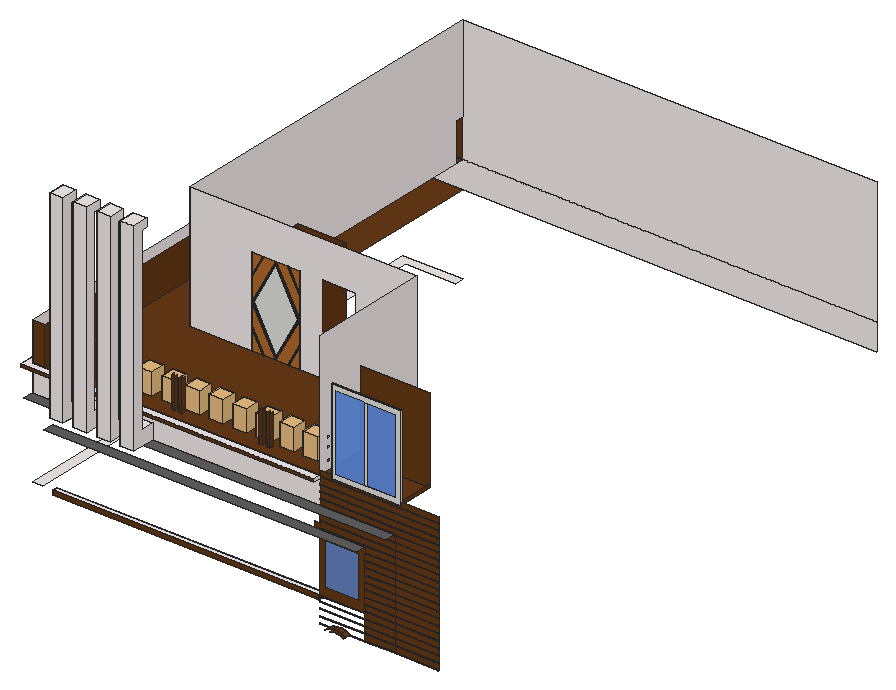
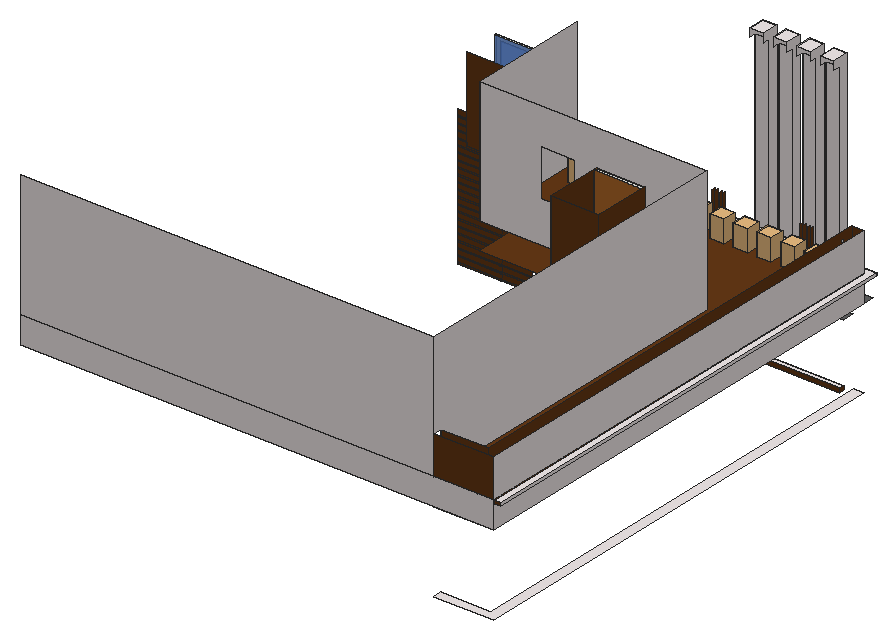
# SketchUp Ruby script. Lengths in inches.
U = 1.inch
M = Sketchup.active_model
def pt(a) = Geom::Point3d.new(a.map { |v| v * U })
def face(e, loops, mat)
  f = e.add_face(loops[0].map { |a| pt(a) })
  loops[1..].each { |l| e.add_face(l.map { |a| pt(a) }).erase! }
  f.material = f.back_material = mat if mat
  f
end
# faces: each face lists its corners as indices into pts; further lists are holes
def faces(e, pts, list, mat = nil) = list.each { |f| face(e, (f[0].is_a?(Array) ? f : [f]).map { |l| l.map { |i| pts[i] } }, mat) }
# xy, xz, yz: faces in a plane at the given z, y or x. An outline is a flat list of corners, or four numbers for a rectangle; further outlines are holes
def ring(l) = l.size == 4 ? [[l[0], l[1]], [l[2], l[1]], [l[2], l[3]], [l[0], l[3]]] : l.each_slice(2).to_a
def flat(e, list, mat, &to3) = list.each { |f| face(e, (f[0].is_a?(Array) ? f : [f]).map { |l| ring(l).map { |u, v| to3.(u, v) } }, mat) }
def xy(e, z, list, mat = nil) = flat(e, list, mat) { |x, y| [x, y, z] }
def xz(e, y, list, mat = nil) = flat(e, list, mat) { |x, z| [x, y, z] }
def yz(e, x, list, mat = nil) = flat(e, list, mat) { |y, z| [x, y, z] }
def lines(e, pts, list) = list.each { |a, b| e.add_line(pt(pts[a]), pt(pts[b])) }
# prism: a flat outline (further loops are holes) pulled along v
def prism(e, loops, v, mat = nil)
  f = face(e, loops, mat); d = Geom::Vector3d.new(v.map { |x| x * U })
  f.pushpull(f.normal.samedirection?(d) ? d.length : -d.length)
end
def box(e, o, s, mat = nil) = prism(e, [[o, [o[0] + s[0], o[1], o[2]], [o[0] + s[0], o[1] + s[1], o[2]], [o[0], o[1] + s[1], o[2]]]], [0, 0, s[2]], mat)
def at(x, y, z, deg = 0) = Geom::Transformation.translation(pt([x, y, z])) * Geom::Transformation.rotation(ORIGIN, Z_AXIS, deg.degrees)
def axes(o, x, y, z) = Geom::Transformation.new([*x, 0, *y, 0, *z, 0, *pt(o).to_a, 1])
def part(name) = M.definitions.add(name)
# library, detail: a bought-in or finely detailed component or shape, given as its bounding box
def library(name, o, s) = part(name).tap { |d| box(d.entities, o, s) }
def detail(e, o, s) = box(e.add_group.entities, o, s)
def put(e, d, t, mat = nil) = e.add_instance(d, t).tap { |i| i.material = mat if mat }
def group(e, t, mat = nil) = e.add_group.tap { |g| g.transformation = t; g.material = mat if mat }.entities
root = M.entities
M.materials.add("Generic").color = [102, 57, 22]
M.materials.add("Generic\#1").color = [96, 96, 96]
M.materials.add("Generic\#3").color = [243, 235, 235]
M.materials.add("[Color M08]").color = [30, 30, 30]
M.materials.add("[Translucent Glass Blue]").color = [100, 149, 237]
M.materials["[Translucent Glass Blue]"].alpha = 0.79
M.materials.add("[Translucent Glass Blue]1").color = [100, 149, 237]
M.materials["[Translucent Glass Blue]1"].alpha = 0.5
M.materials.add("[Wood Bamboo]").color = [177, 105, 43]
c1 = part("Group\#5")
xy(c1.entities,0,[[0,0,33.5625,3]],"[Wood Bamboo]")
xy(c1.entities,44.875,[[0,0,33.5625,3]],"[Wood Bamboo]")
xz(c1.entities,0,[[3.04,3.04,15.78,41.84],[17.78,3.04,30.53,41.84]],"[Translucent Glass Blue]1")
xz(c1.entities,0,[[[0,0,33.5625,44.875],[3.04,3.04,15.78,41.84],[17.78,3.04,30.53,41.84]]],"[Wood Bamboo]")
xz(c1.entities,3,[[0,0,33.5625,44.875]],"[Translucent Glass Blue]1")
yz(c1.entities,0,[[0,0,3,44.875]],"[Wood Bamboo]")
yz(c1.entities,33.5625,[[0,0,3,44.875]],"[Wood Bamboo]")
c2 = part("Group\#3")
xy(c2.entities,14.5,[[0,9,13.0625,22.4375]])
xy(c2.entities,193.75,[[0,0,13.0625,15.5]])
xz(c2.entities,0,[[0,0,13.0625,193.75]])
xz(c2.entities,9,[[0,14.5,13.0625,185.625]])
yz(c2.entities,0,[[0,0,0,193.75,15.5,193.75,15.5,185.625,9,185.625,9,14.5,22.4375,14.5,22.4375,0]])
yz(c2.entities,13.0625,[[0,0,22.4375,0,22.4375,14.5,9,14.5,9,185.625,15.5,185.625,15.5,193.75,0,193.75]])
c3 = library("Raised potted plant",[1.65,0,0],[13.63,13.63,20.73])
c4 = part("Group\#4")
xy(c4.entities,0,[[10.55,0,10.55,0.4375,0,0.4375,0,3.4375,46.1875,3.4375,46.1875,0.4375,35.64,0.4375,35.64,0,34.64,0,34.64,0.4375,11.55,0.4375,11.55,0]])
xy(c4.entities,84.6875,[[11,0,11.55,0,11.55,0.4375,34.64,0.4375,34.64,0,35.1875,0,35.1875,0.4375,46.1875,0.4375,46.1875,3.4375,0,3.4375,0,0.4375,11,0.4375]])
xz(c4.entities,0,[[10.55,0,11.55,0,0,21.17,0,19.34],[[23.09,0,46.1875,42.34,23.09,84.6875,0,42.34],[23.09,2.875,1.57,42.34,23.09,81.8125,44.62,42.34]],[34.64,0,35.64,0,46.1875,19.34,46.1875,21.17],[0,63.52,11.55,84.6875,11,84.6875,0,64.52],[46.1875,63.52,46.1875,64.52,35.1875,84.6875,34.64,84.6875]],"[Color M08]")
xz(c4.entities,0.4375,[[23.09,2.875,44.62,42.34,23.09,81.8125,1.57,42.34]])
xz(c4.entities,0.4375,[[0,0,10.55,0,0,19.34],[11.55,0,23.09,0,0,42.34,0,21.17],[23.09,0,34.64,0,46.1875,21.17,46.1875,42.34],[35.64,0,46.1875,0,46.1875,19.34],[0,42.34,23.09,84.6875,11.55,84.6875,0,63.52],
  [46.1875,42.34,46.1875,63.52,34.64,84.6875,23.09,84.6875],[0,64.52,11,84.6875,0,84.6875],[46.1875,64.52,46.1875,84.6875,35.1875,84.6875]],"[Wood Bamboo]")
xz(c4.entities,3.4375,[[0,0,46.1875,84.6875]],"[Wood Bamboo]")
yz(c4.entities,0,[[0.4375,0,0.4375,19.34,0,19.34,0,21.17,0.4375,21.17,0.4375,63.52,0,63.52,0,64.52,0.4375,64.52,0.4375,84.6875,3.4375,84.6875,3.4375,0]],"[Wood Bamboo]")
yz(c4.entities,46.1875,[[0.4375,0,3.4375,0,3.4375,84.6875,0.4375,84.6875,0.4375,64.52,0,64.52,0,63.52,0.4375,63.52,0.4375,21.17,0,21.17,0,19.34,0.4375,19.34]],"[Wood Bamboo]")
p = [[0,0.4375,19.34],[10.55,0.4375,0],[10.55,0,0],[0,0,19.34],[0,0.4375,42.34],[23.09,0.4375,0],
  [23.09,0,0],[0,0,42.34],[11.55,0.4375,0],[0,0.4375,21.17],[0,0,21.17],[11.55,0,0],
  [46.1875,0.4375,42.34],[46.1875,0,42.34],[46.1875,0.4375,21.17],[34.64,0.4375,0],[34.64,0,0],[46.1875,0,21.17],
  [35.64,0.4375,0],[46.1875,0.4375,19.34],[46.1875,0,19.34],[35.64,0,0],[23.09,0.4375,2.875],[1.57,0.4375,42.34],
  [1.57,0,42.34],[23.09,0,2.875],[44.62,0.4375,42.34],[44.62,0,42.34],[23.09,0.4375,84.6875],[23.09,0,84.6875],
  [23.09,0.4375,81.8125],[23.09,0,81.8125],[0,0.4375,63.52],[11.55,0.4375,84.6875],[11.55,0,84.6875],[0,0,63.52],
  [34.64,0.4375,84.6875],[46.1875,0.4375,63.52],[46.1875,0,63.52],[34.64,0,84.6875],[11,0.4375,84.6875],[0,0.4375,64.52],
  [0,0,64.52],[11,0,84.6875],[46.1875,0.4375,64.52],[35.1875,0.4375,84.6875],[35.1875,0,84.6875],[46.1875,0,64.52]]
faces(c4.entities,p,[[0,1,2,3],[4,5,6,7],[8,9,10,11],[5,12,13,6],[14,15,16,17],[18,19,20,21],[22,23,24,25],[26,22,25,27],
  [28,4,7,29],[23,30,31,24],[12,28,29,13],[30,26,27,31],[32,33,34,35],[36,37,38,39],[40,41,42,43],[44,45,46,47]],"[Color M08]")
xy(root,163.4375,[[360.31,54.375,403,54.68]],"Generic")
xy(root,164.4375,[[360.31,54.375,403,54.68]],"Generic")
xy(root,169.75,[[360.31,54.375,403,54.68]],"Generic")
xy(root,170.75,[[360.31,54.375,403,54.68]],"Generic")
xy(root,176.0625,[[360.31,54.375,403,54.68]],"Generic")
xy(root,177.0625,[[360.31,54.375,403,54.68]],"Generic")
xy(root,182.375,[[360.31,54.375,403,54.68]],"Generic")
xy(root,183.375,[[360.31,54.375,403,54.68]],"Generic")
xy(root,184.5625,[[32.25,54.375,288.56,59.625]],"Generic")
xy(root,185.5625,[[196.46,171.5,230.03,208.375]],"Generic")
xy(root,188.375,[[288.56,53.375,331.74,54.375]],"Generic")
xy(root,188.375,[[32.25,54.375,288.56,59.625]],"Generic\#3")
xy(root,188.56,[[13.1875,54.375,22.72,54.375,22.72,489.875,70.5625,489.875,70.5625,498.375,13.1875,498.375]],"Generic\#3")
xy(root,188.6875,[[360.31,54.375,403,54.68]],"Generic")
xy(root,189.6875,[[360.31,54.375,403,54.68]],"Generic")
xy(root,195,[[360.31,54.375,403,54.68]],"Generic")
xy(root,196,[[360.31,54.375,403,54.68]],"Generic")
xy(root,201.3125,[[360.31,54.375,403,54.68]],"Generic")
xy(root,202.3125,[[360.31,54.375,403,54.68]],"Generic")
xy(root,207.625,[[360.31,54.375,403,54.68]],"Generic")
xy(root,208.625,[[360.31,54.375,403,54.68]],"Generic")
xy(root,213.9375,[[360.31,54.375,403,54.68]],"Generic")
xy(root,214.9375,[[360.31,54.375,403,54.68]],"Generic")
xy(root,220.25,[[360.31,54.375,403,54.68]],"Generic")
xy(root,221.25,[[360.31,54.375,403,54.68]],"Generic")
xy(root,226.5625,[[360.31,54.375,403,54.68]],"Generic")
xy(root,227.5625,[[360.31,54.375,403,54.68]],"Generic")
xy(root,230.4375,[[129.97,171.5,176.16,226.25],[196.46,171.5,230.03,208.375]],"Generic")
xy(root,232.875,[[360.31,54.375,403,54.68]],"Generic")
xy(root,233.875,[[360.31,54.375,403,54.68]],"Generic")
xy(root,239.1875,[[360.31,54.375,403,54.68]],"Generic")
xy(root,240.1875,[[360.31,54.375,403,54.68]],"Generic")
xy(root,245.11,[[32.25,43.5625,331.74,54.375]],"Generic\#1")
xy(root,245.5,[[360.31,54.375,403,54.68]],"Generic")
xy(root,246.5,[[360.31,54.375,403,54.68]],"Generic")
xy(root,251.8125,[[360.31,54.375,403,54.68]],"Generic")
xy(root,252.8125,[[360.31,54.375,403,54.68]],"Generic")
xy(root,258.125,[[360.31,54.375,403,54.68]],"Generic")
xy(root,259.125,[[360.31,54.375,403,54.68]],"Generic")
xy(root,264.4375,[[360.31,54.375,403,54.68]],"Generic")
xy(root,265.4375,[[360.31,54.375,403,54.68]],"Generic")
xy(root,265.75,[[47.2,31.9375,60.27,43.5625],[47.2,43.5625,60.27,54.375],[13.1875,54.375,288.56,171.5],[13.1875,171.5,70.5625,498.375]],"Generic")
xy(root,265.75,[[13.1875,43.5625,47.2,54.375],[60.27,43.5625,360.31,54.375]],"Generic\#1")
xy(root,270.75,[[288.56,54.375,403,54.68]],"Generic")
xy(root,271.75,[[288.56,54.375,403,54.68]],"Generic")
xy(root,277.0625,[[288.56,54.375,403,54.68]],"Generic")
xy(root,278.0625,[[288.56,54.375,403,54.68]],"Generic")
xy(root,283.375,[[288.56,54.375,377.375,54.68],[377.375,54.375,403,54.68]],"Generic")
xy(root,284.375,[[288.56,54.375,377.375,54.68],[377.375,54.375,403,54.68]],"Generic")
xy(root,288.5,[[6.6875,47.4375,6.6875,498.375,13.1875,498.375,13.1875,54.375,288.56,54.375,288.56,47.4375]],"Generic")
xy(root,289.6875,[[288.56,54.375,377.375,54.68],[377.375,54.375,403,54.68]],"Generic")
xy(root,290.6875,[[288.56,54.375,377.375,54.68],[377.375,54.375,403,54.68]],"Generic")
xy(root,291.5,[[13.1875,54.375,13.1875,498.375,70.5625,498.375,70.5625,490.0625,25.02,490.0625,25.02,54.375],[[25.02,54.375,25.02,490.0625,70.5625,490.0625,70.5625,171.5,129.97,171.5,129.97,226.25,176.16,226.25,176.16,171.5,288.56,171.5,288.56,54.375,64.75,54.375,64.75,66.56,61.68,66.56,61.68,54.375],[230.56,63.57,233.62,66.56],[54.37,63.57,57.43,66.56],[138.81,63.57,141.87,66.56],[146.12,63.57,149.18,66.56],[223.25,63.57,226.31,66.56]],[61.68,54.375,64.75,63.57],[54.37,63.57,57.43,66.56],[61.68,63.57,64.75,66.56],
  [138.81,63.57,141.87,66.56],[146.12,63.57,149.18,66.56],[223.25,63.57,226.31,66.56],[230.56,63.57,233.62,66.56]],"Generic")
xy(root,291.5,[[6.6875,47.4375,288.56,47.4375,288.56,54.375,13.1875,54.375,13.1875,498.375,6.6875,498.375]],"Generic\#3")
xy(root,292.6,[[299.81,54.375,366.12,89.74]],"Generic")
xz(root,47.4375,[[6.6875,288.5,288.56,291.5]],"Generic")
xz(root,54.375,[[288.56,163.4375,331.74,164.4375],[331.74,163.4375,360.31,164.4375],[331.74,164.4375,360.31,169.75],[360.31,164.4375,403,169.75],[288.56,169.75,331.74,170.75],
  [331.74,169.75,360.31,170.75],[331.74,170.75,360.31,176.0625],[360.31,170.75,403,176.0625],[288.56,176.0625,331.74,177.0625],[331.74,176.0625,360.31,177.0625],
  [331.74,177.0625,360.31,182.375],[360.31,177.0625,403,182.375],[288.56,182.375,331.74,183.375],[331.74,182.375,360.31,183.375],[331.74,183.375,360.31,188.6875],
  [360.31,183.375,403,188.6875],[32.25,184.5625,288.56,188.375],[288.56,188.375,331.74,245.11],[331.74,188.6875,360.31,189.6875],[331.74,189.6875,360.31,195],
  [360.31,189.6875,403,195],[331.74,195,360.31,196],[331.74,196,360.31,201.3125],[360.31,196,403,201.3125],[331.74,201.3125,360.31,202.3125],
  [331.74,202.3125,360.31,207.625],[360.31,202.3125,403,207.625],[331.74,207.625,360.31,208.625],[331.74,208.625,360.31,213.9375],[360.31,208.625,403,213.9375],
  [331.74,213.9375,360.31,214.9375],[331.74,214.9375,360.31,220.25],[360.31,214.9375,403,220.25],[331.74,220.25,360.31,221.25],[331.74,221.25,360.31,226.5625],
  [360.31,221.25,403,226.5625],[331.74,226.5625,360.31,227.5625],[331.74,227.5625,360.31,232.875],[360.31,227.5625,403,232.875],[331.74,232.875,360.31,233.875],
  [331.74,233.875,360.31,239.1875],[360.31,233.875,403,239.1875],[331.74,239.1875,360.31,240.1875],[331.74,240.1875,360.31,240.1875,360.31,245.5,288.56,245.5,288.56,245.11,331.74,245.11],[360.31,240.1875,403,245.5],
  [284.06,245.11,288.56,250.86],[288.56,245.5,360.31,246.5],[288.56,246.5,360.31,251.8125],[360.31,246.5,403,251.8125],[288.56,251.8125,360.31,252.8125],
  [288.56,252.8125,360.31,258.125],[360.31,252.8125,403,258.125],[288.56,258.125,360.31,259.125],[288.56,259.125,360.31,264.4375],[360.31,259.125,403,264.4375],
  [288.56,264.4375,360.31,265.4375],[288.56,265.4375,360.31,265.75],[360.31,265.4375,403,265.4375,403,270.75,288.56,270.75,288.56,265.75,360.31,265.75],[288.56,270.75,403,271.75],[288.56,271.75,403,277.0625],
  [288.56,277.0625,403,278.0625],[288.56,278.0625,403,283.375],[288.56,284.375,403,289.6875],[13.1875,288.5,288.56,291.5],[288.56,290.6875,403,290.6875,403,296,366.12,296,366.12,292.6,299.81,292.6,299.81,296,288.56,296],
  [13.1875,291.5,25.02,328.375]],"Generic")
xz(root,54.375,[[13.1875,265.75,47.2,265.75,47.2,280.25,60.27,280.25,60.27,265.75,288.56,265.75,288.56,288.5,13.1875,288.5]],"Generic\#3")
xz(root,54.68,[[360.31,163.4375,403,164.4375],[360.31,169.75,403,170.75],[360.31,176.0625,403,177.0625],[360.31,182.375,403,183.375],[360.31,188.6875,403,189.6875],
  [360.31,195,403,196],[360.31,201.3125,403,202.3125],[360.31,207.625,403,208.625],[360.31,213.9375,403,214.9375],[360.31,220.25,403,221.25],
  [360.31,226.5625,403,227.5625],[360.31,232.875,403,233.875],[360.31,239.1875,403,240.1875],[360.31,245.5,403,246.5],[360.31,251.8125,403,252.8125],
  [360.31,258.125,403,259.125],[360.31,264.4375,403,265.4375],[288.56,270.75,403,271.75],[288.56,277.0625,403,278.0625],[288.56,283.375,403,284.375],
  [288.56,289.6875,403,290.6875]],"Generic")
xz(root,59.625,[[32.25,184.5625,288.56,188.375]],"Generic")
xz(root,63.57,[[54.37,291.5,57.43,301.19],[61.68,291.5,64.75,301.19],[138.81,291.5,141.87,298.26],[146.12,291.5,149.18,298.26],[223.25,291.5,226.31,298.26],
  [230.56,291.5,233.62,298.26]],"Generic")
xz(root,66.56,[[54.37,291.5,57.43,298.23],[61.68,291.5,64.75,298.23],[138.81,291.5,141.87,298.23],[146.12,291.5,149.18,298.23],[223.25,291.5,226.31,298.23],
  [230.56,291.5,233.62,298.23]],"Generic")
xz(root,89.74,[[299.81,292.6,366.12,373.92]],"Generic")
xz(root,171.5,[[[70.5625,291.5,129.97,291.5,129.97,376.1875,176.16,376.1875,176.16,291.5,288.56,291.5,288.56,411.5,70.5625,411.5],[196.46,331.3125,230.03,376.1875]]],"Generic\#3")
xz(root,208.375,[[196.46,185.5625,230.03,230.4375]],"Generic")
xz(root,226.25,[[129.97,291.5,176.16,376.1875]],"Generic")
xz(root,490.0625,[[25.02,291.5,70.5625,328.375]],"Generic")
xz(root,498.375,[[6.6875,288.5,13.1875,291.5],[13.1875,291.5,70.5625,328.375]],"Generic")
xz(root,498.375,[[13.1875,265.75,467.875,291.5],[70.5625,291.5,467.875,411.5]],"Generic\#3")
yz(root,6.6875,[[47.4375,288.5,498.375,291.5]],"Generic\#3")
yz(root,13.1875,[[54.375,288.5,498.375,291.5]],"Generic")
yz(root,13.1875,[[54.375,265.75,498.375,288.5],[54.375,291.5,498.375,328.375]],"Generic\#3")
yz(root,25.02,[[[54.375,291.5,490.0625,328.375],[66.56,318.36,63.57,318.38,63.57,321.32,66.56,321.29],[66.56,309.79,63.57,309.82,63.57,312.76,66.56,312.73],[66.56,298.23,63.57,298.26,63.57,301.19,66.56,301.17]]],"Generic")
yz(root,32.25,[[54.375,184.5625,59.625,188.375]],"Generic")
yz(root,54.37,[[63.57,291.5,66.56,321.29]],"Generic")
yz(root,57.43,[[63.57,291.5,66.56,321.29]],"Generic")
yz(root,61.68,[[63.57,291.5,66.56,321.32]],"Generic")
yz(root,64.75,[[63.57,291.5,66.56,321.32]],"Generic")
yz(root,70.5625,[[171.5,291.5,171.5,411.5,498.375,411.5,498.375,328.375,490.0625,328.375,490.0625,291.5]],"Generic\#3")
yz(root,129.97,[[171.5,291.5,226.25,376.1875]],"Generic")
yz(root,138.81,[[63.57,291.5,66.56,321.29]],"Generic")
yz(root,141.87,[[63.57,291.5,66.56,321.29]],"Generic")
yz(root,146.12,[[63.57,291.5,66.56,321.29]],"Generic")
yz(root,149.18,[[63.57,291.5,66.56,321.29]],"Generic")
yz(root,176.16,[[171.5,291.5,226.25,376.1875]],"Generic")
yz(root,196.46,[[171.5,185.5625,208.375,230.4375]],"Generic")
yz(root,223.25,[[63.57,291.5,66.56,321.32]],"Generic")
yz(root,226.31,[[63.57,291.5,66.56,321.32]],"Generic")
yz(root,230.03,[[171.5,185.5625,208.375,230.4375]],"Generic")
yz(root,230.56,[[63.57,291.5,66.56,321.32]],"Generic")
yz(root,233.62,[[63.57,291.5,66.56,321.32]],"Generic")
yz(root,288.56,[[53.375,184.5625,54.375,188.375],[54.375,184.5625,59.625,188.375],[54.375,270.75,54.68,271.75],[54.375,277.0625,54.68,278.0625],[54.375,283.375,54.68,284.375],
  [54.375,289.6875,54.68,290.6875]],"Generic")
yz(root,288.56,[[47.4375,288.5,54.375,291.5],[[54.375,291.5,54.375,378.0625,54.68,378.0625,54.68,379.0625,54.375,379.0625,54.375,384.375,54.68,384.375,54.68,385.375,54.375,385.375,54.375,390.6875,54.68,390.6875,54.68,391.6875,54.375,391.6875,54.375,397,54.68,397,54.68,398,54.375,398,54.375,403.3125,54.68,403.3125,54.68,404.3125,54.375,404.3125,54.375,409.625,54.68,409.625,54.68,410.625,54.375,410.625,54.375,411.5,171.5,411.5,171.5,291.5],[66.56,318.36,66.56,321.29,63.57,321.32,63.57,318.38],[66.56,309.79,66.56,312.73,63.57,312.76,63.57,309.82],[66.56,298.23,66.56,301.17,63.57,301.19,63.57,298.26]]],"Generic\#3")
yz(root,299.81,[[54.375,292.6,89.74,296]],"Generic")
yz(root,360.31,[[54.375,163.4375,54.68,164.4375],[54.375,169.75,54.68,170.75],[54.375,176.0625,54.68,177.0625],[54.375,182.375,54.68,183.375],[54.375,188.6875,54.68,189.6875],
  [54.375,195,54.68,196],[54.375,201.3125,54.68,202.3125],[54.375,207.625,54.68,208.625],[54.375,213.9375,54.68,214.9375],[54.375,220.25,54.68,221.25],
  [54.375,226.5625,54.68,227.5625],[54.375,232.875,54.68,233.875],[54.375,239.1875,54.68,240.1875],[54.375,245.5,54.68,246.5],[54.375,251.8125,54.68,252.8125],
  [54.375,258.125,54.68,259.125],[54.375,264.4375,54.68,265.4375]],"Generic")
yz(root,366.12,[[54.375,292.6,89.74,296]],"Generic")
yz(root,403,[[54.375,163.4375,54.68,164.4375],[54.375,169.75,54.68,170.75],[54.375,176.0625,54.68,177.0625],[54.375,182.375,54.68,183.375],[54.375,188.6875,54.68,189.6875],
  [54.375,195,54.68,196],[54.375,201.3125,54.68,202.3125],[54.375,207.625,54.68,208.625],[54.375,213.9375,54.68,214.9375],[54.375,220.25,54.68,221.25],
  [54.375,226.5625,54.68,227.5625],[54.375,232.875,54.68,233.875],[54.375,239.1875,54.68,240.1875],[54.375,245.5,54.68,246.5],[54.375,251.8125,54.68,252.8125],
  [54.375,258.125,54.68,259.125],[54.375,264.4375,54.68,265.4375],[54.375,270.75,54.68,271.75],[54.375,277.0625,54.68,278.0625],[54.375,283.375,54.68,284.375],
  [54.375,289.6875,54.68,290.6875]],"Generic")
p = [[314.1,53.375,165.08],[317.23,53.375,163.4],[317.23,47.75,163.4],[314.1,47.75,165.08],[302.7,53.375,166.93],[299.15,53.375,164.73],
  [299.15,47.75,164.73],[302.7,47.75,166.93],[303.6875,53.375,164.75],[307.09,53.375,165.78],[307.09,47.75,165.78],[303.6875,47.75,164.75],
  [310.64,53.375,165.89],[310.64,47.75,165.89],[318.625,53.375,165.34],[314.94,53.375,167.31],[314.94,47.75,167.31],[318.625,47.75,165.34],
  [306.7,53.375,168.14],[306.7,47.75,168.14],[310.88,53.375,168.27],[310.88,47.75,168.27],[315,56.0625,291.5],[315,54.375,291.5],
  [318.06,56.0625,291.5],[310.75,56.0625,291.5],[307.68,56.0625,291.5]]
faces(root,p,[[0,1,2,3],[4,5,6,7],[8,9,10,11],[12,0,3,13],[14,15,16,17],[9,12,13,10],[18,4,7,19],[15,20,21,16],
  [20,18,19,21]],"Generic")
lines(root,p,[[22,23],[24,22],[25,26]])
put(root,c1,at(196.46,171.5,185.5625))
g1 = group(root,at(288.56,54.375,188.375))
xz(g1,0,[[[0,0,43.1875,56.73],[6.03,7.86,37.15,48.87]]])
xz(g1,0,[[6.03,7.86,37.15,48.87]],"[Translucent Glass Blue]")
put(root,c2,at(69.83,31.9375,265.75),"Generic\#3")
put(root,c2,at(92.45,31.9375,265.75),"Generic\#3")
put(root,c2,at(115.08,31.9375,265.75),"Generic\#3")
put(root,c2,at(47.2,31.9375,265.75),"Generic\#3")
put(root,c3,at(258.45,70.3125,291.5))
put(root,c3,at(235.76,70.3125,291.5))
put(root,c3,at(213.08,70.3125,291.5))
put(root,c3,at(190.39,70.3125,291.5))
put(root,c3,at(167.7,70.3125,291.5))
put(root,c3,at(145.01,70.3125,291.5))
put(root,c3,at(122.33,70.3125,291.5))
put(root,c3,at(99.64,70.3125,291.5))
put(root,c3,at(76.95,70.3125,291.5))
put(root,c3,at(54.26,70.3125,291.5))
put(root,c3,at(31.58,70.3125,291.5))
put(root,c4,at(129.97,171.0625,291.5))
g2 = group(root,at(299.81,54.375,292.6))
xy(g2,0,[[0,0,9.36,2],[9.36,0,16.48,2],[16.48,0,66.3125,2]])
xy(g2,81.3125,[[0,0,66.3125,2]])
xz(g2,0,[[[0,0,66.3125,81.3125],[4.61,4.61,61.7,76.7]],[31.66,4.61,34.66,76.7]])
xz(g2,0,[[4.61,4.61,31.66,76.7],[34.66,4.61,61.7,76.7]],"[Translucent Glass Blue]")
xz(g2,2,[[0,0,66.3125,81.3125]],"[Translucent Glass Blue]")
yz(g2,0,[[0,0,2,81.3125]])
yz(g2,66.3125,[[0,0,2,81.3125]])
